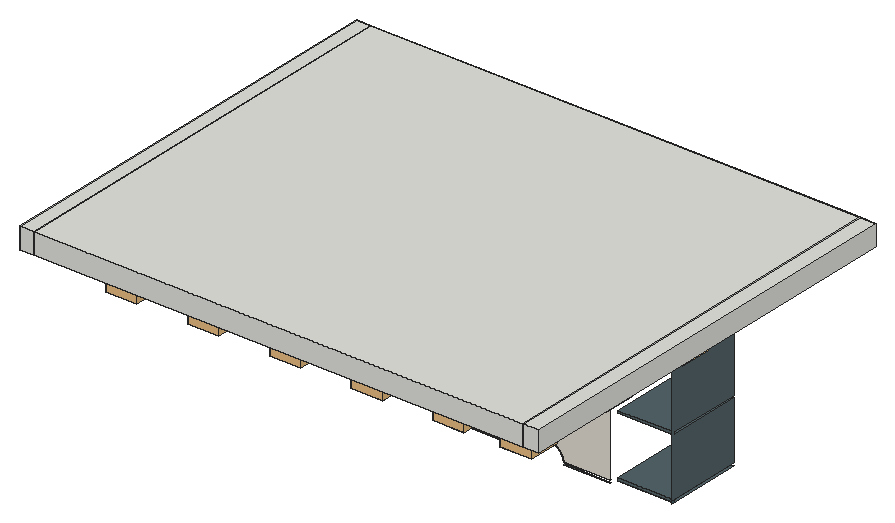
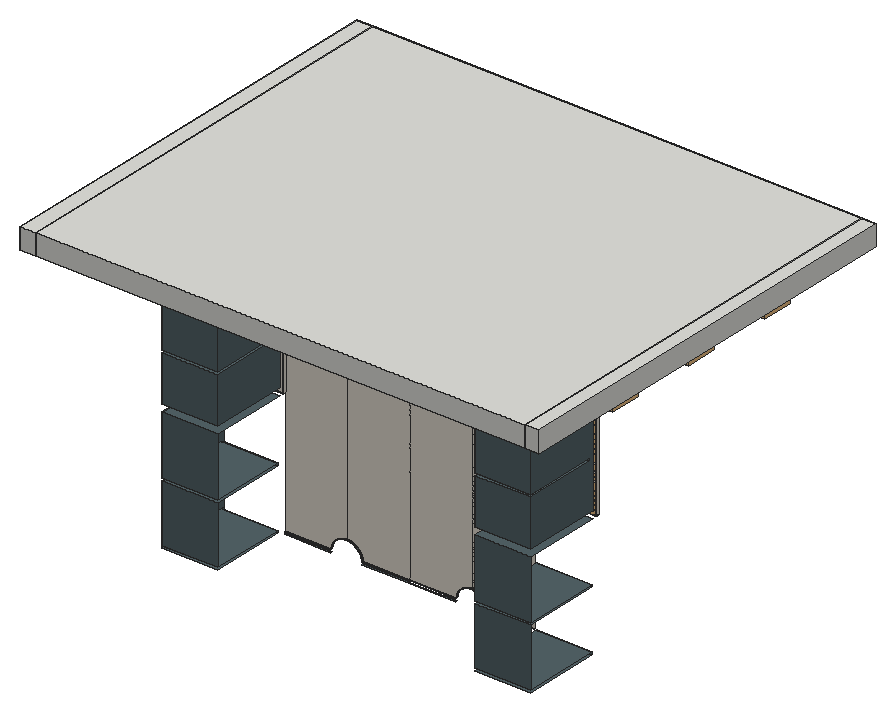
# SketchUp Ruby script. Lengths in millimetres.
U = 1.mm
M = Sketchup.active_model
def pt(a) = Geom::Point3d.new(a.map { |v| v * U })
def face(e, loops, mat)
  f = e.add_face(loops[0].map { |a| pt(a) })
  loops[1..].each { |l| e.add_face(l.map { |a| pt(a) }).erase! }
  f.material = f.back_material = mat if mat
  f
end
# faces: each face lists its corners as indices into pts; further lists are holes
def faces(e, pts, list, mat = nil) = list.each { |f| face(e, (f[0].is_a?(Array) ? f : [f]).map { |l| l.map { |i| pts[i] } }, mat) }
# xy, xz, yz: faces in a plane at the given z, y or x. An outline is a flat list of corners, or four numbers for a rectangle; further outlines are holes
def ring(l) = l.size == 4 ? [[l[0], l[1]], [l[2], l[1]], [l[2], l[3]], [l[0], l[3]]] : l.each_slice(2).to_a
def flat(e, list, mat, &to3) = list.each { |f| face(e, (f[0].is_a?(Array) ? f : [f]).map { |l| ring(l).map { |u, v| to3.(u, v) } }, mat) }
def xy(e, z, list, mat = nil) = flat(e, list, mat) { |x, y| [x, y, z] }
def xz(e, y, list, mat = nil) = flat(e, list, mat) { |x, z| [x, y, z] }
def yz(e, x, list, mat = nil) = flat(e, list, mat) { |y, z| [x, y, z] }
def lines(e, pts, list) = list.each { |a, b| e.add_line(pt(pts[a]), pt(pts[b])) }
# prism: a flat outline (further loops are holes) pulled along v
def prism(e, loops, v, mat = nil)
  f = face(e, loops, mat); d = Geom::Vector3d.new(v.map { |x| x * U })
  f.pushpull(f.normal.samedirection?(d) ? d.length : -d.length)
end
def box(e, o, s, mat = nil) = prism(e, [[o, [o[0] + s[0], o[1], o[2]], [o[0] + s[0], o[1] + s[1], o[2]], [o[0], o[1] + s[1], o[2]]]], [0, 0, s[2]], mat)
def at(x, y, z, deg = 0) = Geom::Transformation.translation(pt([x, y, z])) * Geom::Transformation.rotation(ORIGIN, Z_AXIS, deg.degrees)
def axes(o, x, y, z) = Geom::Transformation.new([*x, 0, *y, 0, *z, 0, *pt(o).to_a, 1])
def part(name) = M.definitions.add(name)
# library, detail: a bought-in or finely detailed component or shape, given as its bounding box
def library(name, o, s) = part(name).tap { |d| box(d.entities, o, s) }
def detail(e, o, s) = box(e.add_group.entities, o, s)
def put(e, d, t, mat = nil) = e.add_instance(d, t).tap { |i| i.material = mat if mat }
def group(e, t, mat = nil) = e.add_group.tap { |g| g.transformation = t; g.material = mat if mat }.entities
root = M.entities
M.materials.add("Olon-Denim-Chic-VT14-1K").color = [84, 100, 105]
M.materials.add("Olon-Fresh-Linen-VT10-1K").color = [226, 220, 209]
M.materials.add("Pionite-a-Panolam-Brand-Tidal-Pool-SB045-4K").color = [68, 97, 103]
c1 = part("Group\#3")
detail(c1.entities,[0,0,0],[453,18,760.5])
c2 = library("Group\#10",[0,0,0],[226.1,226.1,320.6])
c3 = part("Group\#1")
xy(c3.entities,0,[[12.7,0,114.3,3048],[114.3,0,3657.6,3048],[3657.6,0,3771.9,3048]])
xy(c3.entities,152.4,[[12.7,0,114.3,3048],[114.3,0,3657.6,3048],[3657.6,0,3771.9,3048]])
xz(c3.entities,0,[[12.7,0,114.3,152.4],[114.3,0,3657.6,152.4],[3657.6,0,3771.9,152.4]])
xz(c3.entities,3048,[[12.7,0,114.3,152.4],[114.3,0,3657.6,152.4],[3657.6,0,3771.9,152.4]])
yz(c3.entities,12.7,[[0,0,3048,152.4]])
yz(c3.entities,114.3,[[0,0,3048,152.4]])
yz(c3.entities,3657.6,[[0,0,3048,152.4]])
yz(c3.entities,3771.9,[[0,0,3048,152.4]])
xy(root,1216.3,[[1171.6,2324.1,1511.3,2333.1],[1514.3,2324.1,1854,2333.1],[2077.5,2324.1,2414.2,2333.1]],"Olon-Denim-Chic-VT14-1K")
xy(root,1225.3,[[177.8,2344.1,580,2904.1],[2442.6,2362.1,2844.8,2904.1]],"Olon-Denim-Chic-VT14-1K")
xy(root,1234.3,[[608.4,2324.1,948.1,2333.1],[1171.6,2324.1,1511.3,2333.1],[1514.3,2324.1,1854,2333.1],[2077.5,2324.1,2414.2,2333.1]],"Olon-Denim-Chic-VT14-1K")
xy(root,1243.3,[[177.8,2344.1,580,2904.1],[2442.6,2362.1,2844.8,2904.1]],"Olon-Denim-Chic-VT14-1K")
xy(root,1662.2,[[177.8,2344.1,580,2904.1],[2442.6,2362.1,2844.8,2904.1]],"Olon-Denim-Chic-VT14-1K")
xy(root,1680.2,[[177.8,2344.1,580,2904.1],[2442.6,2362.1,2844.8,2904.1]],"Olon-Denim-Chic-VT14-1K")
xy(root,2108.2,[[177.8,2342.1,580,2904.1],[2442.6,2342.1,2844.8,2904.1]],"Olon-Denim-Chic-VT14-1K")
xy(root,2159,[[177.8,2342.1,580,2904.1],[2442.6,2342.1,2844.8,2904.1]],"Pionite-a-Panolam-Brand-Tidal-Pool-SB045-4K")
xy(root,2492.9,[[177.8,2364.1,580,2904.1],[2442.6,2364.1,2844.8,2904.1]],"Olon-Denim-Chic-VT14-1K")
xy(root,2510.9,[[177.8,2364.1,580,2904.1],[2442.6,2364.1,2844.8,2904.1]],"Olon-Denim-Chic-VT14-1K")
xy(root,2844.8,[[177.8,2342.1,580,2904.1],[2442.6,2342.1,2844.8,2904.1]],"Olon-Denim-Chic-VT14-1K")
xy(root,2895.6,[[101.6,2324.1,149.4,2324.1,149.4,2342.1,152.4,2342.1,152.4,2933.7,101.6,2933.7],[608.4,2324.1,1058.3,2324.1,1058.3,2342.1,1061.3,2342.1,1061.3,2324.1,1511.3,2324.1,1511.3,2342.1,1514.3,2342.1,1514.3,2324.1,1964.3,2324.1,1964.3,2342.1,1967.3,2342.1,1967.3,2324.1,2414.2,2324.1,2414.2,2342.1,2870.2,2342.1,2870.2,2933.7,152.4,2933.7,152.4,2342.1,608.4,2342.1],[2873.2,2324.1,2921,2324.1,2921,2933.7,2870.2,2933.7,2870.2,2342.1,2873.2,2342.1]],"Olon-Fresh-Linen-VT10-1K")
xz(root,2324.1,[[608.4,1234.3,948.1,1234.3,948.2,1235.7,948.6,1239.1,949.1,1242.6,949.7,1246,950.4,1249.4,951.2,1252.8,952.1,1256.1,953.1,1259.4,955.5,1266,956.8,1269.2,958.3,1272.4,959.8,1275.5,961.4,1278.5,963.1,1281.6,966.9,1287.4,968.9,1290.3,970.9,1293.1,973.1,1295.8,977.7,1301,980.1,1303.5,982.6,1305.9,987.8,1310.5,990.5,1312.7,993.3,1314.7,996.2,1316.7,1002,1320.5,1005.1,1322.2,1008.1,1323.8,1011.2,1325.3,1014.4,1326.8,1017.6,1328.1,1020.9,1329.3,1027.5,1331.5,1030.8,1332.4,1034.2,1333.2,1037.6,1333.9,1041,1334.5,1044.5,1335,1047.9,1335.4,1054.9,1335.8,1058.3,1335.9,1058.3,2895.6,608.4,2895.6],[1171.6,1234.3,1511.3,1234.3,1511.3,2895.6,1061.3,2895.6,1061.3,1335.9,1064.8,1335.8,1068.3,1335.6,1071.7,1335.4,1075.2,1335,1078.6,1334.5,1082.1,1333.9,1085.5,1333.2,1088.8,1332.4,1092.2,1331.5,1098.8,1329.3,1102,1328.1,1105.3,1326.8,1111.5,1323.8,1114.6,1322.2,1117.6,1320.5,1120.6,1318.6,1123.5,1316.7,1129.1,1312.7,1131.8,1310.5,1134.5,1308.2,1137,1305.9,1139.5,1303.5,1142,1301,1146.6,1295.8,1148.7,1293.1,1150.8,1290.3,1152.8,1287.4,1154.7,1284.5,1156.5,1281.6,1158.3,1278.5,1159.9,1275.5,1161.4,1272.4,1164.2,1266,1165.4,1262.7,1166.5,1259.4,1168.5,1252.8,1169.3,1249.4,1170,1246,1170.6,1242.6,1171.1,1239.1,1171.4,1235.7],[1514.3,1234.3,1854,1234.3,1854.2,1235.7,1854.5,1239.1,1855,1242.6,1855.6,1246,1856.3,1249.4,1857.1,1252.8,1859.1,1259.4,1860.2,1262.7,1861.4,1266,1864.2,1272.4,1865.7,1275.5,1867.3,1278.5,1869.1,1281.6,1870.9,1284.5,1872.8,1287.4,1874.8,1290.3,1876.9,1293.1,1879,1295.8,1883.6,1301,1886.1,1303.5,1888.6,1305.9,1891.1,1308.2,1893.8,1310.5,1896.5,1312.7,1902.1,1316.7,1905,1318.6,1908,1320.5,1911,1322.2,1914.1,1323.8,1920.3,1326.8,1923.6,1328.1,1926.8,1329.3,1933.4,1331.5,1936.8,1332.4,1940.1,1333.2,1943.5,1333.9,1947,1334.5,1950.4,1335,1953.9,1335.4,1957.3,1335.6,1960.8,1335.8,1964.3,1335.9,1964.3,2895.6,1514.3,2895.6],[2077.5,1234.3,2414.2,1234.3,2414.2,2895.6,1967.3,2895.6,1967.3,1335.9,1970.7,1335.8,1977.7,1335.4,1981.1,1335,1984.6,1334.5,1988,1333.9,1991.4,1333.2,1994.8,1332.4,1998.1,1331.5,2004.7,1329.3,2008,1328.1,2011.2,1326.8,2014.4,1325.3,2017.5,1323.8,2020.5,1322.2,2023.6,1320.5,2029.4,1316.7,2032.3,1314.7,2035.1,1312.7,2037.8,1310.5,2043,1305.9,2045.5,1303.5,2047.9,1301,2052.5,1295.8,2054.7,1293.1,2056.7,1290.3,2058.7,1287.4,2062.5,1281.6,2064.2,1278.5,2065.8,1275.5,2067.3,1272.4,2068.8,1269.2,2070.1,1266,2072.5,1259.4,2073.5,1256.1,2074.4,1252.8,2075.2,1249.4,2075.9,1246,2076.5,1242.6,2077,1239.1,2077.4,1235.7]],"Olon-Fresh-Linen-VT10-1K")
xz(root,2342.1,[[152.4,2132.1,605.4,2135.1],[2417.2,2132.1,2870.2,2135.1],[[152.4,2135.1,605.4,2895.6],[177.8,2159,580,2844.8]],[[2417.2,2135.1,2870.2,2895.6],[2442.6,2159,2844.8,2844.8]]],"Olon-Fresh-Linen-VT10-1K")
xz(root,2344.1,[[177.8,1225.3,580,1243.3],[177.8,1662.2,580,1680.2]],"Olon-Denim-Chic-VT14-1K")
xz(root,2362.1,[[2442.6,1225.3,2844.8,1243.3],[2442.6,1662.2,2844.8,1680.2]],"Olon-Denim-Chic-VT14-1K")
xz(root,2364.1,[[177.8,2492.9,580,2510.9],[2442.6,2492.9,2844.8,2510.9]],"Olon-Denim-Chic-VT14-1K")
xz(root,2904.1,[[177.8,1243.3,580,1662.2],[2442.6,1243.3,2844.8,1662.2],[177.8,1680.2,580,2108.2],[2442.6,1680.2,2844.8,2108.2],[177.8,2159,580,2492.9],
  [2442.6,2159,2844.8,2492.9],[177.8,2510.9,580,2844.8],[2442.6,2510.9,2844.8,2844.8]],"Olon-Denim-Chic-VT14-1K")
yz(root,149.4,[[2324.1,2132.1,2342.1,2135.1],[2324.1,2135.1,2342.1,2895.6]],"Olon-Fresh-Linen-VT10-1K")
yz(root,177.8,[[2342.1,2159,2904.1,2159,2904.1,2492.9,2364.1,2492.9,2364.1,2510.9,2904.1,2510.9,2904.1,2844.8,2342.1,2844.8]],"Olon-Denim-Chic-VT14-1K")
yz(root,580,[[2342.1,2159,2342.1,2844.8,2904.1,2844.8,2904.1,2510.9,2364.1,2510.9,2364.1,2492.9,2904.1,2492.9,2904.1,2159]],"Olon-Denim-Chic-VT14-1K")
yz(root,608.4,[[2324.1,2132.1,2342.1,2135.1],[2324.1,2135.1,2342.1,2895.6]],"Olon-Fresh-Linen-VT10-1K")
yz(root,2414.2,[[2324.1,2133.6,2342.1,2895.6]],"Olon-Fresh-Linen-VT10-1K")
yz(root,2442.6,[[2342.1,2159,2904.1,2159,2904.1,2492.9,2364.1,2492.9,2364.1,2510.9,2904.1,2510.9,2904.1,2844.8,2342.1,2844.8]],"Olon-Denim-Chic-VT14-1K")
yz(root,2844.8,[[2342.1,1243.3,2342.1,2108.2,2904.1,2108.2,2904.1,1680.2,2362.1,1680.2,2362.1,1662.2,2904.1,1662.2,2904.1,1243.3],[2342.1,2159,2342.1,2844.8,2904.1,2844.8,2904.1,2510.9,2364.1,2510.9,2364.1,2492.9,2904.1,2492.9,2904.1,2159]],"Olon-Denim-Chic-VT14-1K")
yz(root,2844.8,[[2342.1,1225.3,2362.1,1243.3]],"Pionite-a-Panolam-Brand-Tidal-Pool-SB045-4K")
yz(root,2873.2,[[2324.1,2133.6,2342.1,2895.6]],"Olon-Fresh-Linen-VT10-1K")
p = [[948.2,2324.1,1235.7],[948.1,2324.1,1234.3],[948.1,2333.1,1234.3],[948.2,2333.1,1235.7],[1171.6,2324.1,1234.3],[1171.4,2324.1,1235.7],
  [1171.4,2333.1,1235.7],[1171.6,2333.1,1234.3],[1854.2,2324.1,1235.7],[1854,2324.1,1234.3],[1854,2333.1,1234.3],[1854.2,2333.1,1235.7],
  [2077.5,2324.1,1234.3],[2077.4,2324.1,1235.7],[2077.4,2333.1,1235.7],[2077.5,2333.1,1234.3],[948.6,2324.1,1239.1],[948.6,2333.1,1239.1],
  [1171.1,2324.1,1239.1],[1171.1,2333.1,1239.1],[1854.5,2324.1,1239.1],[1854.5,2333.1,1239.1],[2077,2324.1,1239.1],[2077,2333.1,1239.1],
  [949.1,2324.1,1242.6],[949.1,2333.1,1242.6],[1170.6,2324.1,1242.6],[1170.6,2333.1,1242.6],[1855,2324.1,1242.6],[1855,2333.1,1242.6],
  [2076.5,2324.1,1242.6],[2076.5,2333.1,1242.6],[949.7,2324.1,1246],[949.7,2333.1,1246],[1170,2324.1,1246],[1170,2333.1,1246],
  [1855.6,2324.1,1246],[1855.6,2333.1,1246],[2075.9,2324.1,1246],[2075.9,2333.1,1246],[950.4,2324.1,1249.4],[950.4,2333.1,1249.4],
  [1169.3,2324.1,1249.4],[1169.3,2333.1,1249.4],[1856.3,2324.1,1249.4],[1856.3,2333.1,1249.4],[2075.2,2324.1,1249.4],[2075.2,2333.1,1249.4],
  [951.2,2324.1,1252.8],[951.2,2333.1,1252.8],[1168.5,2324.1,1252.8],[1168.5,2333.1,1252.8],[1857.1,2324.1,1252.8],[1857.1,2333.1,1252.8],
  [2074.4,2324.1,1252.8],[2074.4,2333.1,1252.8],[952.1,2324.1,1256.1],[952.1,2333.1,1256.1],[1167.5,2324.1,1256.1],[1167.5,2333.1,1256.1],
  [1858.1,2324.1,1256.1],[1858.1,2333.1,1256.1],[2073.5,2324.1,1256.1],[2073.5,2333.1,1256.1],[953.1,2324.1,1259.4],[953.1,2333.1,1259.4],
  [1166.5,2324.1,1259.4],[1166.5,2333.1,1259.4],[1859.1,2324.1,1259.4],[1859.1,2333.1,1259.4],[2072.5,2324.1,1259.4],[2072.5,2333.1,1259.4],
  [954.3,2324.1,1262.7],[954.3,2333.1,1262.7],[1165.4,2324.1,1262.7],[1165.4,2333.1,1262.7],[1860.2,2324.1,1262.7],[1860.2,2333.1,1262.7],
  [2071.3,2324.1,1262.7],[2071.3,2333.1,1262.7],[955.5,2324.1,1266],[955.5,2333.1,1266],[1164.2,2324.1,1266],[1164.2,2333.1,1266],
  [1861.4,2324.1,1266],[1861.4,2333.1,1266],[2070.1,2324.1,1266],[2070.1,2333.1,1266],[956.8,2324.1,1269.2],[956.8,2333.1,1269.2],
  [1162.8,2324.1,1269.2],[1162.8,2333.1,1269.2],[1862.8,2324.1,1269.2],[1862.8,2333.1,1269.2],[2068.8,2324.1,1269.2],[2068.8,2333.1,1269.2],
  [958.3,2324.1,1272.4],[958.3,2333.1,1272.4],[1161.4,2324.1,1272.4],[1161.4,2333.1,1272.4],[1864.2,2324.1,1272.4],[1864.2,2333.1,1272.4],
  [2067.3,2324.1,1272.4],[2067.3,2333.1,1272.4],[959.8,2324.1,1275.5],[959.8,2333.1,1275.5],[1159.9,2324.1,1275.5],[1159.9,2333.1,1275.5],
  [1865.7,2324.1,1275.5],[1865.7,2333.1,1275.5],[2065.8,2324.1,1275.5],[2065.8,2333.1,1275.5],[961.4,2324.1,1278.5],[961.4,2333.1,1278.5],
  [1158.3,2324.1,1278.5],[1158.3,2333.1,1278.5],[1867.3,2324.1,1278.5],[1867.3,2333.1,1278.5],[2064.2,2324.1,1278.5],[2064.2,2333.1,1278.5],
  [963.1,2324.1,1281.6],[963.1,2333.1,1281.6],[1156.5,2324.1,1281.6],[1156.5,2333.1,1281.6],[1869.1,2324.1,1281.6],[1869.1,2333.1,1281.6],
  [2062.5,2324.1,1281.6],[2062.5,2333.1,1281.6],[965,2324.1,1284.5],[965,2333.1,1284.5],[1154.7,2324.1,1284.5],[1154.7,2333.1,1284.5],
  [1870.9,2324.1,1284.5],[1870.9,2333.1,1284.5],[2060.6,2324.1,1284.5],[2060.6,2333.1,1284.5],[966.9,2324.1,1287.4],[966.9,2333.1,1287.4],
  [1152.8,2324.1,1287.4],[1152.8,2333.1,1287.4],[1872.8,2324.1,1287.4],[1872.8,2333.1,1287.4],[2058.7,2324.1,1287.4],[2058.7,2333.1,1287.4],
  [968.9,2324.1,1290.3],[968.9,2333.1,1290.3],[1150.8,2324.1,1290.3],[1150.8,2333.1,1290.3],[1874.8,2324.1,1290.3],[1874.8,2333.1,1290.3],
  [2056.7,2324.1,1290.3],[2056.7,2333.1,1290.3],[970.9,2324.1,1293.1],[970.9,2333.1,1293.1],[1148.7,2324.1,1293.1],[1148.7,2333.1,1293.1],
  [1876.9,2324.1,1293.1],[1876.9,2333.1,1293.1],[2054.7,2324.1,1293.1],[2054.7,2333.1,1293.1],[973.1,2324.1,1295.8],[973.1,2333.1,1295.8],
  [1146.6,2324.1,1295.8],[1146.6,2333.1,1295.8],[1879,2324.1,1295.8],[1879,2333.1,1295.8],[2052.5,2324.1,1295.8],[2052.5,2333.1,1295.8],
  [975.4,2324.1,1298.4],[975.4,2333.1,1298.4],[1144.3,2324.1,1298.4],[1144.3,2333.1,1298.4],[1881.3,2324.1,1298.4],[1881.3,2333.1,1298.4],
  [2050.2,2324.1,1298.4],[2050.2,2333.1,1298.4],[977.7,2324.1,1301],[977.7,2333.1,1301],[1142,2324.1,1301],[1142,2333.1,1301],
  [1883.6,2324.1,1301],[1883.6,2333.1,1301],[2047.9,2324.1,1301],[2047.9,2333.1,1301],[980.1,2324.1,1303.5],[980.1,2333.1,1303.5],
  [1139.5,2324.1,1303.5],[1139.5,2333.1,1303.5],[1886.1,2324.1,1303.5],[1886.1,2333.1,1303.5],[2045.5,2324.1,1303.5],[2045.5,2333.1,1303.5],
  [982.6,2324.1,1305.9],[982.6,2333.1,1305.9],[1137,2324.1,1305.9],[1137,2333.1,1305.9],[1888.6,2324.1,1305.9],[1888.6,2333.1,1305.9],
  [2043,2324.1,1305.9],[2043,2333.1,1305.9],[985.2,2324.1,1308.2],[985.2,2333.1,1308.2],[1134.5,2324.1,1308.2],[1134.5,2333.1,1308.2],
  [1891.1,2324.1,1308.2],[1891.1,2333.1,1308.2],[2040.4,2324.1,1308.2],[2040.4,2333.1,1308.2],[987.8,2324.1,1310.5],[987.8,2333.1,1310.5],
  [1131.8,2324.1,1310.5],[1131.8,2333.1,1310.5],[1893.8,2324.1,1310.5],[1893.8,2333.1,1310.5],[2037.8,2324.1,1310.5],[2037.8,2333.1,1310.5],
  [990.5,2324.1,1312.7],[990.5,2333.1,1312.7],[1129.1,2324.1,1312.7],[1129.1,2333.1,1312.7],[1896.5,2324.1,1312.7],[1896.5,2333.1,1312.7],
  [2035.1,2324.1,1312.7],[2035.1,2333.1,1312.7],[993.3,2324.1,1314.7],[993.3,2333.1,1314.7],[1126.3,2324.1,1314.7],[1126.3,2333.1,1314.7],
  [1899.3,2324.1,1314.7],[1899.3,2333.1,1314.7],[2032.3,2324.1,1314.7],[2032.3,2333.1,1314.7],[996.2,2324.1,1316.7],[996.2,2333.1,1316.7],
  [1123.5,2324.1,1316.7],[1123.5,2333.1,1316.7],[1902.1,2324.1,1316.7],[1902.1,2333.1,1316.7],[2029.4,2324.1,1316.7],[2029.4,2333.1,1316.7],
  [999.1,2324.1,1318.6],[999.1,2333.1,1318.6],[1120.6,2324.1,1318.6],[1120.6,2333.1,1318.6],[1905,2324.1,1318.6],[1905,2333.1,1318.6],
  [2026.5,2324.1,1318.6],[2026.5,2333.1,1318.6],[1002,2324.1,1320.5],[1002,2333.1,1320.5],[1117.6,2324.1,1320.5],[1117.6,2333.1,1320.5],
  [1908,2324.1,1320.5],[1908,2333.1,1320.5],[2023.6,2324.1,1320.5],[2023.6,2333.1,1320.5],[1005.1,2324.1,1322.2],[1005.1,2333.1,1322.2],
  [1114.6,2324.1,1322.2],[1114.6,2333.1,1322.2],[1911,2324.1,1322.2],[1911,2333.1,1322.2],[2020.5,2324.1,1322.2],[2020.5,2333.1,1322.2],
  [1008.1,2324.1,1323.8],[1008.1,2333.1,1323.8],[1111.5,2324.1,1323.8],[1111.5,2333.1,1323.8],[1914.1,2324.1,1323.8],[1914.1,2333.1,1323.8],
  [2017.5,2324.1,1323.8],[2017.5,2333.1,1323.8],[1011.2,2324.1,1325.3],[1011.2,2333.1,1325.3],[1108.4,2324.1,1325.3],[1108.4,2333.1,1325.3],
  [1917.2,2324.1,1325.3],[1917.2,2333.1,1325.3],[2014.4,2324.1,1325.3],[2014.4,2333.1,1325.3],[1014.4,2324.1,1326.8],[1014.4,2333.1,1326.8],
  [1105.3,2324.1,1326.8],[1105.3,2333.1,1326.8],[1920.3,2324.1,1326.8],[1920.3,2333.1,1326.8],[2011.2,2324.1,1326.8],[2011.2,2333.1,1326.8],
  [1017.6,2324.1,1328.1],[1017.6,2333.1,1328.1],[1102,2324.1,1328.1],[1102,2333.1,1328.1],[1923.6,2324.1,1328.1],[1923.6,2333.1,1328.1],
  [2008,2324.1,1328.1],[2008,2333.1,1328.1],[1020.9,2324.1,1329.3],[1020.9,2333.1,1329.3],[1098.8,2324.1,1329.3],[1098.8,2333.1,1329.3],
  [1926.8,2324.1,1329.3],[1926.8,2333.1,1329.3],[2004.7,2324.1,1329.3],[2004.7,2333.1,1329.3],[1024.2,2324.1,1330.4],[1024.2,2333.1,1330.4],
  [1095.5,2324.1,1330.4],[1095.5,2333.1,1330.4],[1930.1,2324.1,1330.4],[1930.1,2333.1,1330.4],[2001.4,2324.1,1330.4],[2001.4,2333.1,1330.4],
  [1027.5,2324.1,1331.5],[1027.5,2333.1,1331.5],[1092.2,2324.1,1331.5],[1092.2,2333.1,1331.5],[1933.4,2324.1,1331.5],[1933.4,2333.1,1331.5],
  [1998.1,2324.1,1331.5],[1998.1,2333.1,1331.5],[1030.8,2324.1,1332.4],[1030.8,2333.1,1332.4],[1088.8,2324.1,1332.4],[1088.8,2333.1,1332.4],
  [1936.8,2324.1,1332.4],[1936.8,2333.1,1332.4],[1994.8,2324.1,1332.4],[1994.8,2333.1,1332.4],[1034.2,2324.1,1333.2],[1034.2,2333.1,1333.2],
  [1085.5,2324.1,1333.2],[1085.5,2333.1,1333.2],[1940.1,2324.1,1333.2],[1940.1,2333.1,1333.2],[1991.4,2324.1,1333.2],[1991.4,2333.1,1333.2],
  [1037.6,2324.1,1333.9],[1037.6,2333.1,1333.9],[1082.1,2324.1,1333.9],[1082.1,2333.1,1333.9],[1943.5,2324.1,1333.9],[1943.5,2333.1,1333.9],
  [1988,2324.1,1333.9],[1988,2333.1,1333.9],[1041,2324.1,1334.5],[1041,2333.1,1334.5],[1078.6,2324.1,1334.5],[1078.6,2333.1,1334.5],
  [1947,2324.1,1334.5],[1947,2333.1,1334.5],[1984.6,2324.1,1334.5],[1984.6,2333.1,1334.5],[1044.5,2324.1,1335],[1044.5,2333.1,1335],
  [1075.2,2324.1,1335],[1075.2,2333.1,1335],[1950.4,2324.1,1335],[1950.4,2333.1,1335],[1981.1,2324.1,1335],[1981.1,2333.1,1335],
  [1047.9,2324.1,1335.4],[1047.9,2333.1,1335.4],[1071.7,2324.1,1335.4],[1071.7,2333.1,1335.4],[1953.9,2324.1,1335.4],[1953.9,2333.1,1335.4],
  [1977.7,2324.1,1335.4],[1977.7,2333.1,1335.4],[1051.4,2324.1,1335.6],[1051.4,2333.1,1335.6],[1068.3,2324.1,1335.6],[1068.3,2333.1,1335.6],
  [1957.3,2324.1,1335.6],[1957.3,2333.1,1335.6],[1974.2,2324.1,1335.6],[1974.2,2333.1,1335.6],[1054.9,2324.1,1335.8],[1054.9,2333.1,1335.8],
  [1064.8,2324.1,1335.8],[1064.8,2333.1,1335.8],[1960.8,2324.1,1335.8],[1960.8,2333.1,1335.8],[1970.7,2324.1,1335.8],[1970.7,2333.1,1335.8],
  [1058.3,2324.1,1335.9],[1058.3,2333.1,1335.9],[1061.3,2324.1,1335.9],[1061.3,2333.1,1335.9],[1964.3,2324.1,1335.9],[1964.3,2333.1,1335.9],
  [1967.3,2324.1,1335.9],[1967.3,2333.1,1335.9]]
faces(root,p,[[0,1,2,3],[4,5,6,7],[8,9,10,11],[12,13,14,15],[16,0,3,17],[5,18,19,6],[20,8,11,21],[13,22,23,14],
  [24,16,17,25],[18,26,27,19],[28,20,21,29],[22,30,31,23],[32,24,25,33],[26,34,35,27],[36,28,29,37],[30,38,39,31],
  [40,32,33,41],[34,42,43,35],[44,36,37,45],[38,46,47,39],[48,40,41,49],[42,50,51,43],[52,44,45,53],[46,54,55,47],
  [56,48,49,57],[50,58,59,51],[60,52,53,61],[54,62,63,55],[64,56,57,65],[58,66,67,59],[68,60,61,69],[62,70,71,63],
  [72,64,65,73],[66,74,75,67],[76,68,69,77],[70,78,79,71],[80,72,73,81],[74,82,83,75],[84,76,77,85],[78,86,87,79],
  [88,80,81,89],[82,90,91,83],[92,84,85,93],[86,94,95,87],[96,88,89,97],[90,98,99,91],[100,92,93,101],[94,102,103,95],
  [104,96,97,105],[98,106,107,99],[108,100,101,109],[102,110,111,103],[112,104,105,113],[106,114,115,107],[116,108,109,117],[110,118,119,111],
  [120,112,113,121],[114,122,123,115],[124,116,117,125],[118,126,127,119],[128,120,121,129],[122,130,131,123],[132,124,125,133],[126,134,135,127],
  [136,128,129,137],[130,138,139,131],[140,132,133,141],[134,142,143,135],[144,136,137,145],[138,146,147,139],[148,140,141,149],[142,150,151,143],
  [152,144,145,153],[146,154,155,147],[156,148,149,157],[150,158,159,151],[160,152,153,161],[154,162,163,155],[164,156,157,165],[158,166,167,159],
  [168,160,161,169],[162,170,171,163],[172,164,165,173],[166,174,175,167],[176,168,169,177],[170,178,179,171],[180,172,173,181],[174,182,183,175],
  [184,176,177,185],[178,186,187,179],[188,180,181,189],[182,190,191,183],[192,184,185,193],[186,194,195,187],[196,188,189,197],[190,198,199,191],
  [200,192,193,201],[194,202,203,195],[204,196,197,205],[198,206,207,199],[208,200,201,209],[202,210,211,203],[212,204,205,213],[206,214,215,207],
  [216,208,209,217],[210,218,219,211],[220,212,213,221],[214,222,223,215],[224,216,217,225],[218,226,227,219],[228,220,221,229],[222,230,231,223],
  [232,224,225,233],[226,234,235,227],[236,228,229,237],[230,238,239,231],[240,232,233,241],[234,242,243,235],[244,236,237,245],[238,246,247,239],
  [248,240,241,249],[242,250,251,243],[252,244,245,253],[246,254,255,247],[256,248,249,257],[250,258,259,251],[260,252,253,261],[254,262,263,255],
  [264,256,257,265],[258,266,267,259],[268,260,261,269],[262,270,271,263],[272,264,265,273],[266,274,275,267],[276,268,269,277],[270,278,279,271],
  [280,272,273,281],[274,282,283,275],[284,276,277,285],[278,286,287,279],[288,280,281,289],[282,290,291,283],[292,284,285,293],[286,294,295,287],
  [296,288,289,297],[290,298,299,291],[300,292,293,301],[294,302,303,295],[304,296,297,305],[298,306,307,299],[308,300,301,309],[302,310,311,303],
  [312,304,305,313],[306,314,315,307],[316,308,309,317],[310,318,319,311],[320,312,313,321],[314,322,323,315],[324,316,317,325],[318,326,327,319],
  [328,320,321,329],[322,330,331,323],[332,324,325,333],[326,334,335,327],[336,328,329,337],[330,338,339,331],[340,332,333,341],[334,342,343,335],
  [344,336,337,345],[338,346,347,339],[348,340,341,349],[342,350,351,343],[352,344,345,353],[346,354,355,347],[356,348,349,357],[350,358,359,351],
  [360,352,353,361],[354,362,363,355],[364,356,357,365],[358,366,367,359],[368,360,361,369],[362,370,371,363],[372,364,365,373],[366,374,375,367],
  [376,368,369,377],[370,378,379,371],[380,372,373,381],[374,382,383,375],[384,376,377,385],[378,386,387,379],[388,380,381,389],[382,390,391,383]],"Olon-Denim-Chic-VT14-1K")
put(root,c1,at(152.4,2324.1,2135.1),"Olon-Fresh-Linen-VT10-1K")
put(root,c1,at(2417.2,2324.1,2135.1),"Olon-Fresh-Linen-VT10-1K")
put(root,c2,at(327.9,1741.2,2581))
put(root,c2,at(920,1741.2,2581))
put(root,c2,at(1512.1,1741.2,2581))
put(root,c2,at(2104.3,1741.2,2581))
put(root,c2,at(2696.4,1741.2,2581))
put(root,c2,at(3182.2,1741.2,2581))
put(root,c2,at(3182.2,1055.4,2581))
put(root,c2,at(1512.1,1055.4,2581))
put(root,c2,at(2104.3,1055.4,2581))
put(root,c2,at(2696.4,1055.4,2581))
put(root,c2,at(920,1055.4,2581))
put(root,c2,at(327.9,1055.4,2581))
put(root,c2,at(3182.2,369.6,2581))
put(root,c2,at(1512.1,369.6,2581))
put(root,c2,at(2104.3,369.6,2581))
put(root,c2,at(2696.4,369.6,2581))
put(root,c2,at(920,369.6,2581))
put(root,c2,at(327.9,369.6,2581))
put(root,c3,at(-12.7,0,2901.6))
